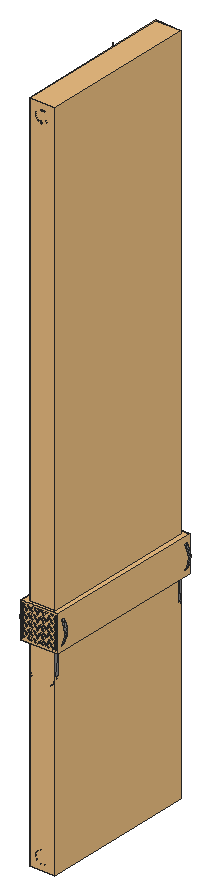
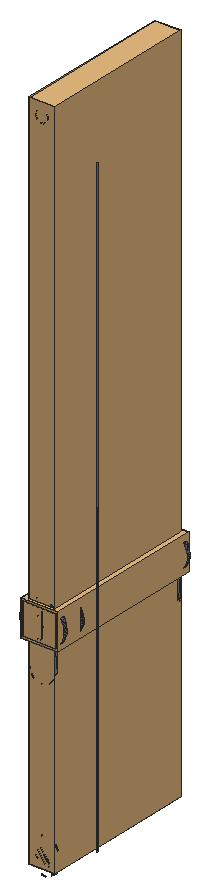
# SketchUp Ruby script. Lengths in inches.
U = 1.inch
M = Sketchup.active_model
def pt(a) = Geom::Point3d.new(a.map { |v| v * U })
def face(e, loops, mat)
  f = e.add_face(loops[0].map { |a| pt(a) })
  loops[1..].each { |l| e.add_face(l.map { |a| pt(a) }).erase! }
  f.material = f.back_material = mat if mat
  f
end
# faces: each face lists its corners as indices into pts; further lists are holes
def faces(e, pts, list, mat = nil) = list.each { |f| face(e, (f[0].is_a?(Array) ? f : [f]).map { |l| l.map { |i| pts[i] } }, mat) }
# xy, xz, yz: faces in a plane at the given z, y or x. An outline is a flat list of corners, or four numbers for a rectangle; further outlines are holes
def ring(l) = l.size == 4 ? [[l[0], l[1]], [l[2], l[1]], [l[2], l[3]], [l[0], l[3]]] : l.each_slice(2).to_a
def flat(e, list, mat, &to3) = list.each { |f| face(e, (f[0].is_a?(Array) ? f : [f]).map { |l| ring(l).map { |u, v| to3.(u, v) } }, mat) }
def xy(e, z, list, mat = nil) = flat(e, list, mat) { |x, y| [x, y, z] }
def xz(e, y, list, mat = nil) = flat(e, list, mat) { |x, z| [x, y, z] }
def yz(e, x, list, mat = nil) = flat(e, list, mat) { |y, z| [x, y, z] }
def lines(e, pts, list) = list.each { |a, b| e.add_line(pt(pts[a]), pt(pts[b])) }
# prism: a flat outline (further loops are holes) pulled along v
def prism(e, loops, v, mat = nil)
  f = face(e, loops, mat); d = Geom::Vector3d.new(v.map { |x| x * U })
  f.pushpull(f.normal.samedirection?(d) ? d.length : -d.length)
end
def box(e, o, s, mat = nil) = prism(e, [[o, [o[0] + s[0], o[1], o[2]], [o[0] + s[0], o[1] + s[1], o[2]], [o[0], o[1] + s[1], o[2]]]], [0, 0, s[2]], mat)
def at(x, y, z, deg = 0) = Geom::Transformation.translation(pt([x, y, z])) * Geom::Transformation.rotation(ORIGIN, Z_AXIS, deg.degrees)
def axes(o, x, y, z) = Geom::Transformation.new([*x, 0, *y, 0, *z, 0, *pt(o).to_a, 1])
def part(name) = M.definitions.add(name)
# library, detail: a bought-in or finely detailed component or shape, given as its bounding box
def library(name, o, s) = part(name).tap { |d| box(d.entities, o, s) }
def detail(e, o, s) = box(e.add_group.entities, o, s)
def put(e, d, t, mat = nil) = e.add_instance(d, t).tap { |i| i.material = mat if mat }
def group(e, t, mat = nil) = e.add_group.tap { |g| g.transformation = t; g.material = mat if mat }.entities
root = M.entities
M.materials.add("Material \#1").color = [140, 140, 140]
c1 = library("3DGeom~4_Defintion",[-18.02,-499.97,-221.16],[36.04,1000,262.12])
c2 = part("3DGeom~5_Defintion")
xy(c2.entities,-225.24,[[-0.79,-499.98,-2.33,-499.64,7.45,-496.14],[-0.79,-499.98,7.45,-496.14,1.58,-499.88],[1.58,-499.88,7.45,-496.14,3.84,-499.16],[-2.33,-499.64,7.4,-485.75,7.45,-496.14],[3.84,-499.16,7.45,-496.14,5.85,-497.89],
  [7.45,-496.14,7.4,-485.75,8.24,-487.08],[7.45,-496.14,8.24,-487.08,8.96,-489.34],[7.45,-496.14,8.96,-489.34,9.0625,-491.71],[7.45,-496.14,9.0625,-491.71,8.55,-494.03],[-7.4,-496.08,-8.24,-494.76,2.32,-482.2],
  [-8.24,-494.76,-8.96,-492.5,2.32,-482.2],[-8.96,-492.5,-9.0625,-490.125,2.32,-482.2],[-9.0625,-490.125,-8.55,-487.81,2.32,-482.2],[-8.55,-487.81,-7.45,-485.7,2.32,-482.2],[-7.45,-485.7,-5.85,-483.95,2.32,-482.2],
  [-5.85,-483.95,-3.84,-482.68,2.32,-482.2],[-3.84,-482.68,-1.58,-481.96,2.32,-482.2],[2.32,-482.2,-1.58,-481.96,0.79,-481.86],[0,481.82,-2.35,482.13,-6.92,496.71],[0,481.82,-6.92,496.71,1.55,482.04],
  [-2.35,482.13,-4.55,483.04,-6.92,496.71],[-4.55,483.04,-6.43,484.49,-6.92,496.71],[-6.43,484.49,-7.88,486.37,-6.92,496.71],[6.92,485.12,-1.55,499.8125,7.88,495.47],[6.92,485.12,7.88,495.47,7.88,486.37],
  [-7.88,486.37,-8.79,488.57,-6.92,496.71],[7.88,486.37,7.88,495.47,8.79,488.57],[-8.79,488.57,-9.1,490.92,-6.92,496.71],[8.79,488.57,7.88,495.47,9.1,490.92],[-9.1,490.92,-8.79,493.28,-6.92,496.71],
  [9.1,490.92,7.88,495.47,8.79,493.28],[-8.79,493.28,-7.88,495.47,-6.92,496.71],[7.88,495.47,-1.55,499.8125,0,500.02],[7.88,495.47,0,500.02,2.35,499.71],[7.88,495.47,2.35,499.71,4.55,498.8],
  [7.88,495.47,4.55,498.8,6.43,497.35]],"Material \#1")
xy(c2.entities,-221.57,[[-2.33,-499.64,-5.22,-498.37,7.4,-485.75],[-5.22,-498.37,-7.4,-496.08,5.22,-483.47],[-5.22,-498.37,5.22,-483.47,7.4,-485.75],[-7.4,-496.08,2.32,-482.2,5.22,-483.47],[1.55,482.04,-6.92,496.71,-4.55,498.8],
  [1.55,482.04,-4.55,498.8,4.55,483.04],[4.55,483.04,-4.55,498.8,-1.55,499.8125],[4.55,483.04,-1.55,499.8125,6.92,485.12]],"Material \#1")
xy(c2.entities,38.05,[[-2.33,-499.64,7.4,-485.75,-5.22,-498.37],[-5.22,-498.37,5.22,-483.47,-7.4,-496.08],[-5.22,-498.37,7.4,-485.75,5.22,-483.47],[-7.4,-496.08,5.22,-483.47,2.32,-482.2],[1.55,482.04,-4.55,498.8,-6.92,496.71],
  [1.55,482.04,4.55,483.04,-4.55,498.8],[4.55,483.04,-1.55,499.8125,-4.55,498.8],[4.55,483.04,6.92,485.12,-1.55,499.8125]],"Material \#1")
xy(c2.entities,41.72,[[-0.79,-499.98,7.45,-496.14,-2.33,-499.64],[-0.79,-499.98,1.58,-499.88,7.45,-496.14],[1.58,-499.88,3.84,-499.16,7.45,-496.14],[-2.33,-499.64,7.45,-496.14,7.4,-485.75],[3.84,-499.16,5.85,-497.89,7.45,-496.14],
  [7.45,-496.14,8.24,-487.08,7.4,-485.75],[7.45,-496.14,8.55,-494.03,9.0625,-491.71],[7.45,-496.14,8.96,-489.34,8.24,-487.08],[7.45,-496.14,9.0625,-491.71,8.96,-489.34],[-7.4,-496.08,2.32,-482.2,-8.24,-494.76],
  [-8.24,-494.76,2.32,-482.2,-8.96,-492.5],[-8.96,-492.5,2.32,-482.2,-9.0625,-490.125],[-9.0625,-490.125,2.32,-482.2,-8.55,-487.81],[-8.55,-487.81,2.32,-482.2,-7.45,-485.7],[-7.45,-485.7,2.32,-482.2,-5.85,-483.95],
  [-5.85,-483.95,2.32,-482.2,-3.84,-482.68],[-3.84,-482.68,2.32,-482.2,-1.58,-481.96],[2.32,-482.2,0.79,-481.86,-1.58,-481.96],[0,481.82,-6.92,496.71,-2.35,482.13],[0,481.82,1.55,482.04,-6.92,496.71],
  [-2.35,482.13,-6.92,496.71,-4.55,483.04],[-4.55,483.04,-6.92,496.71,-6.43,484.49],[-6.43,484.49,-6.92,496.71,-7.88,486.37],[6.92,485.12,7.88,495.47,-1.55,499.8125],[6.92,485.12,7.88,486.37,7.88,495.47],
  [-7.88,486.37,-6.92,496.71,-8.79,488.57],[7.88,486.37,8.79,488.57,7.88,495.47],[-8.79,488.57,-6.92,496.71,-9.1,490.92],[8.79,488.57,9.1,490.92,7.88,495.47],[-9.1,490.92,-6.92,496.71,-8.79,493.28],
  [9.1,490.92,8.79,493.28,7.88,495.47],[-8.79,493.28,-6.92,496.71,-7.88,495.47],[7.88,495.47,0,500.02,-1.55,499.8125],[7.88,495.47,2.35,499.71,0,500.02],[7.88,495.47,4.55,498.8,2.35,499.71],
  [7.88,495.47,6.43,497.35,4.55,498.8]],"Material \#1")
c3 = part("3DGeom~10_Defintion")
yz(c3.entities,-68.96,[[-797.08,-844.83,-797.08,-827.59,-922.41,-827.59],[-922.41,-844.83,-797.08,-844.83,-922.41,-827.59]],"Material \#1")
yz(c3.entities,68.97,[[-922.41,-844.83,-797.08,-827.59,-797.08,-844.83],[-922.41,-844.83,-922.41,-827.59,-797.08,-827.59],[-797.08,137.93,-922.41,155.17,-797.08,155.17],[-922.41,137.93,-922.41,155.17,-797.08,137.93]],"Material \#1")
p = [[-15.8,-989.55,-844.83],[-15.8,-989.55,-827.59],[0,-991.38,-827.59],[0,-991.38,-844.83],[15.8,-989.55,-827.59],[15.8,-989.55,-844.83],
  [-30.32,-984.36,-844.83],[-30.32,-984.36,-827.59],[30.31,-984.36,-827.59],[30.31,-984.36,-844.83],[-43.12,-976.21,-844.83],[-43.12,-976.21,-827.59],
  [43.12,-976.21,-827.59],[43.12,-976.21,-844.83],[-53.81,-965.53,-844.83],[-53.81,-965.53,-827.59],[53.8,-965.53,-827.59],[53.8,-965.53,-844.83],
  [-61.95,-952.73,-844.83],[-61.95,-952.73,-827.59],[53.8,-965.53,-827.59],[61.95,-952.73,-827.59],[61.95,-952.73,-844.83],[-67.15,-938.21,-844.83],
  [-67.15,-938.21,-827.59],[67.14,-938.21,-827.59],[67.14,-938.21,-844.83],[-68.96,-922.41,-844.83],[-68.96,-922.41,-827.59],[67.14,-938.21,-827.59],
  [68.97,-922.41,-827.59],[68.97,-922.41,-844.83],[-69.1,-794.86,-844.83],[-69.1,-794.86,-827.59],[-68.96,-797.08,-827.59],[-68.96,-797.08,-844.83],
  [68.97,-797.08,-844.83],[68.97,-797.08,-827.59],[69.11,-794.71,-827.59],[69.11,-794.71,-844.83],[-69.48,-792.73,-844.83],[-69.48,-792.73,-827.59],
  [69.53,-792.51,-827.59],[69.53,-792.51,-844.83],[-70.14,-790.6875,-844.83],[-70.14,-790.6875,-827.59],[70.24,-790.48,-827.59],[70.24,-790.48,-844.83],
  [-71.08,-788.73,-844.83],[-71.08,-788.73,-827.59],[71.22,-788.57,-827.59],[71.22,-788.57,-844.83],[-72.32,-786.86,-844.83],[-72.32,-786.86,-827.59],
  [72.47,-786.78,-827.59],[72.47,-786.78,-844.83],[-73.8,-785.17,-844.83],[-73.8,-785.17,-827.59],[74,-785.04,-827.59],[74,-785.04,-844.83],
  [-75.96,-783.21,-844.83],[-75.96,-783.21,-827.59],[74,-785.04,-827.59],[75.76,-783.39,-827.59],[75.76,-783.39,-844.83],[86.625,-772.95,-827.59],
  [86.61,-772.96,-844.83],[-86.89,-773.25,-844.83],[-86.89,-773.25,-827.59],[-75.96,-783.21,-844.83],[-96.66,-761.8,-844.83],[-96.66,-761.8,-827.59],
  [86.625,-772.95,-827.59],[86.63,-772.94,-844.83],[86.61,-772.96,-844.83],[86.625,-772.95,-827.59],[86.62,-772.95,-827.59],[86.62,-772.95,-827.59],
  [96.31,-761.375,-827.59],[96.31,-761.375,-844.83],[86.63,-772.94,-844.83],[86.625,-772.95,-827.59],[86.62,-772.95,-827.59],[-104.96,-749.18,-844.83],
  [-104.96,-749.18,-827.59],[-96.66,-761.8,-827.59],[-96.66,-761.8,-844.83],[96.31,-761.375,-827.59],[104.62,-748.77,-827.59],[104.62,-748.77,-844.83],
  [-111.64,-735.52,-844.83],[-111.64,-735.52,-827.59],[111.39,-735.21,-827.59],[111.39,-735.21,-844.83],[-116.49,-721.23,-844.83],[-116.49,-721.23,-827.59],
  [116.4375,-720.78,-827.59],[116.4375,-720.78,-844.83],[-119.64,-705.62,-844.83],[-119.64,-705.62,-827.59],[119.6,-705.57,-827.59],[119.6,-705.57,-844.83],
  [-120.6875,-689.65,-844.83],[-120.6875,-689.65,-827.59],[120.69,-689.65,-827.59],[120.69,-689.65,-844.83],[-117.5,-662,-844.83],[-117.5,-662,-827.59],
  [117.5,-662,-827.59],[117.5,-662,-844.83],[-108.41,-636.61,-844.83],[-108.41,-636.61,-827.59],[117.5,-662,-844.83],[108.41,-636.61,-827.59],
  [108.41,-636.61,-844.83],[-93.91,-613.95,-844.83],[-93.91,-613.95,-827.59],[-108.41,-636.61,-827.59],[108.41,-636.61,-844.83],[94.16,-614.19,-827.59],
  [94.16,-614.19,-844.83],[94.16,-614.19,-827.59],[75.46,-595.5,-827.59],[75.46,-595.5,-844.83],[-75.46,-595.5,-844.83],[-75.46,-595.5,-827.59],
  [-93.91,-613.95,-827.59],[-93.91,-613.95,-827.59],[-93.91,-613.95,-844.83],[-53.05,-581.24,-844.83],[-53.05,-581.24,-827.59],[-75.46,-595.5,-827.59],
  [-75.46,-595.5,-844.83],[53.05,-581.24,-827.59],[53.05,-581.24,-844.83],[-27.65,-572.16,-844.83],[-27.65,-572.16,-827.59],[-53.05,-581.24,-827.59],
  [-53.05,-581.24,-844.83],[27.66,-572.16,-827.59],[27.66,-572.16,-844.83],[0,-568.97,-844.83],[0,-568.97,-827.59],[-27.65,-572.16,-827.59],
  [-27.65,-572.16,-844.83],[0,-568.97,-844.83],[-15.8,-989.55,155.17],[0,-991.38,155.17],[0,-991.38,137.93],[-15.8,-989.55,137.93],
  [15.8,-989.55,155.17],[15.8,-989.55,137.93],[-30.32,-984.36,155.17],[-30.32,-984.36,137.93],[30.31,-984.36,155.17],[30.31,-984.36,137.93],
  [-43.125,-976.22,155.17],[-43.125,-976.22,137.93],[43.12,-976.22,155.17],[43.12,-976.22,137.93],[-53.81,-965.53,155.17],[-53.81,-965.53,137.93],
  [53.8,-965.53,155.17],[53.8,-965.53,137.93],[-61.96,-952.73,155.17],[-61.95,-952.73,137.93],[61.95,-952.73,155.17],[61.95,-952.73,137.93],
  [53.8,-965.53,137.93],[-67.15,-938.21,155.17],[-67.15,-938.21,137.93],[67.14,-938.21,155.17],[67.14,-938.21,137.93],[-68.96,-922.41,155.17],
  [-68.96,-922.41,137.93],[68.97,-922.41,155.17],[68.97,-922.41,137.93],[67.14,-938.21,137.93],[-68.97,-797.08,155.17],[-68.97,-797.08,137.93],
  [-69.1,-794.86,155.17],[-69.1,-794.86,137.93],[68.97,-797.08,155.17],[69.11,-794.71,155.17],[69.11,-794.71,137.93],[68.97,-797.08,137.93],
  [-69.48,-792.73,155.17],[-69.48,-792.73,137.93],[69.53,-792.51,155.17],[69.53,-792.51,137.93],[-70.14,-790.6875,155.17],[-70.14,-790.6875,137.93],
  [70.24,-790.48,155.17],[70.24,-790.48,137.93],[-71.08,-788.73,155.17],[-71.08,-788.73,137.93],[71.22,-788.57,155.17],[71.22,-788.57,137.93],
  [-72.32,-786.86,155.17],[-72.32,-786.86,137.93],[72.47,-786.78,155.17],[72.47,-786.78,137.93],[-73.8,-785.17,155.17],[-73.8,-785.17,137.93],
  [74,-785.04,155.17],[74,-785.04,137.93],[-75.96,-783.21,155.17],[-75.96,-783.21,137.93],[75.76,-783.39,155.17],[75.76,-783.39,137.93],
  [74,-785.04,137.93],[86.61,-772.96,155.17],[86.625,-772.95,137.93],[-86.88,-773.25,155.17],[-75.96,-783.21,155.17],[-86.88,-773.25,137.93],
  [-96.66,-761.8,155.17],[-96.66,-761.8,137.93],[86.63,-772.94,155.17],[86.625,-772.95,137.93],[86.61,-772.96,155.17],[86.62,-772.95,137.93],
  [86.625,-772.95,137.93],[96.31,-761.375,155.17],[96.31,-761.375,137.93],[86.62,-772.95,137.93],[86.63,-772.94,155.17],[86.62,-772.95,137.93],
  [86.625,-772.95,137.93],[-104.96,-749.18,155.17],[-96.66,-761.8,155.17],[-96.66,-761.8,137.93],[-104.96,-749.18,137.93],[104.62,-748.77,155.17],
  [104.62,-748.77,137.93],[96.31,-761.375,137.93],[-111.64,-735.52,155.17],[-111.64,-735.52,137.93],[111.39,-735.21,155.17],[111.39,-735.21,137.93],
  [-116.49,-721.23,155.17],[-116.49,-721.23,137.93],[116.4375,-720.78,155.17],[116.4375,-720.78,137.93],[-119.64,-705.62,155.17],[-119.64,-705.62,137.93],
  [119.6,-705.57,155.17],[119.6,-705.57,137.93],[-120.6875,-689.65,155.17],[-120.6875,-689.65,137.93],[120.69,-689.65,155.17],[120.69,-689.65,137.93],
  [-117.5,-662,155.17],[-117.5,-662,137.93],[117.5,-662,155.17],[117.5,-662,137.93],[-108.41,-636.61,155.17],[-108.41,-636.61,137.93],
  [117.5,-662,155.17],[108.41,-636.61,155.17],[108.41,-636.61,137.93],[-93.91,-613.95,155.17],[-108.41,-636.61,137.93],[-93.91,-613.95,137.93],
  [108.41,-636.61,155.17],[94.16,-614.19,155.17],[94.16,-614.19,137.93],[75.46,-595.5,155.17],[75.46,-595.5,137.93],[94.16,-614.19,137.93],
  [-75.46,-595.5,155.17],[-93.91,-613.95,155.17],[-93.91,-613.95,137.93],[-75.46,-595.5,137.93],[-53.05,-581.24,155.17],[-75.46,-595.5,155.17],
  [-75.46,-595.5,137.93],[-53.05,-581.24,137.93],[53.05,-581.24,155.17],[53.05,-581.24,137.93],[-27.65,-572.16,155.17],[-53.05,-581.24,155.17],
  [-53.05,-581.24,137.93],[-27.65,-572.16,137.93],[27.65,-572.16,155.17],[27.65,-572.16,137.93],[0,-568.97,155.17],[-27.65,-572.16,155.17],
  [-27.65,-572.16,137.93],[0,-568.97,137.93],[0,-568.97,155.17]]
faces(c3.entities,p,[[0,1,2],[2,3,0],[3,2,4],[4,5,3],[6,7,1],[1,0,6],[5,4,8],[8,9,5],
  [10,11,7],[7,6,10],[9,8,12],[12,13,9],[14,15,11],[11,10,14],[13,12,16],[16,17,13],
  [18,19,15],[15,14,18],[17,20,21],[21,22,17],[23,24,19],[19,18,23],[22,21,25],[25,26,22],
  [27,28,24],[24,23,27],[26,29,30],[30,31,26],[32,33,34],[34,35,32],[36,37,38],[38,39,36],
  [40,41,33],[33,32,40],[39,38,42],[42,43,39],[44,45,41],[41,40,44],[43,42,46],[46,47,43],
  [48,49,45],[45,44,48],[47,46,50],[50,51,47],[52,53,49],[49,48,52],[51,50,54],[54,55,51],
  [56,57,53],[53,52,56],[55,54,58],[58,59,55],[60,61,57],[57,56,60],[59,62,63],[63,64,59],
  [64,63,65],[65,66,64],[67,68,61],[61,69,67],[70,71,68],[68,67,70],[72,73,66],[74,75,76],
  [73,77,78],[78,79,73],[80,81,82],[83,84,85],[85,86,83],[79,87,88],[88,89,79],[90,91,84],
  [84,83,90],[89,88,92],[92,93,89],[94,95,91],[91,90,94],[93,92,96],[96,97,93],[98,99,95],
  [95,94,98],[97,96,100],[100,101,97],[102,103,99],[99,98,102],[101,100,104],[104,105,101],[106,107,103],
  [103,102,106],[105,104,108],[108,109,105],[110,111,107],[107,106,110],[112,108,113],[113,114,112],[115,116,117],
  [117,110,115],[118,113,119],[119,120,118],[120,121,122],[122,123,120],[124,125,126],[127,128,124],[129,130,131],
  [131,132,129],[123,122,133],[133,134,123],[135,136,137],[137,138,135],[134,133,139],[139,140,134],[141,142,143],
  [143,144,141],[140,139,142],[142,145,140],[146,147,148],[148,149,146],[147,150,151],[151,148,147],[152,146,149],
  [149,153,152],[150,154,155],[155,151,150],[156,152,153],[153,157,156],[154,158,159],[159,155,154],[160,156,157],
  [157,161,160],[158,162,163],[163,159,158],[164,160,161],[161,165,164],[162,166,167],[167,168,162],[169,164,165],
  [165,170,169],[166,171,172],[172,167,166],[173,169,170],[170,174,173],[171,175,176],[176,177,171],[178,173,174],
  [174,179,178],[180,178,179],[179,181,180],[182,183,184],[184,185,182],[186,180,181],[181,187,186],[183,188,189],
  [189,184,183],[190,186,187],[187,191,190],[188,192,193],[193,189,188],[194,190,191],[191,195,194],[192,196,197],
  [197,193,192],[198,194,195],[195,199,198],[196,200,201],[201,197,196],[202,198,199],[199,203,202],[200,204,205],
  [205,201,200],[206,202,203],[203,207,206],[204,208,209],[209,210,204],[208,211,212],[212,209,208],[213,214,207],
  [207,215,213],[216,213,215],[215,217,216],[211,218,219],[220,221,222],[218,223,224],[224,225,218],[226,227,228],
  [229,230,231],[231,232,229],[223,233,234],[234,235,223],[236,229,232],[232,237,236],[233,238,239],[239,234,233],
  [240,236,237],[237,241,240],[238,242,243],[243,239,238],[244,240,241],[241,245,244],[242,246,247],[247,243,242],
  [248,244,245],[245,249,248],[246,250,251],[251,247,246],[252,248,249],[249,253,252],[250,254,255],[255,251,250],
  [256,252,253],[253,257,256],[258,259,260],[260,255,258],[261,256,262],[262,263,261],[264,265,266],[266,260,264],
  [265,267,268],[268,269,265],[270,271,272],[272,273,270],[274,275,276],[276,277,274],[267,278,279],[279,268,267],
  [280,281,282],[282,283,280],[278,284,285],[285,279,278],[286,287,288],[288,289,286],[284,290,289],[289,285,284]],"Material \#1")
c4 = library("3DGeom~12_Defintion",[-95.68,-755.75,-830.03],[191.36,191.37,1000])
c5 = library("3DGeom~13_Defintion",[-84.91,-744.98,-830.03],[169.82,169.83,1000])
xy(root,190.239,[[338.044,116.355,338.044,116.676,338.08,116.355],[338.08,116.355,338.044,116.676,338.08,116.676]],"Material \#1")
xy(root,190.555,[[338.027,116.355,338.086,116.676,338.027,116.676]],"Material \#1")
xz(root,116.32,[[338.056,189.714,337.988,189.729,338.124,189.729],[338.056,189.714,338.02,189.718,337.988,189.729],[337.988,189.729,337.901,190.151,338.206,189.829],[337.988,189.729,337.906,189.829,337.901,190.151],[337.988,189.729,337.935,189.77,337.906,189.829],
  [337.988,189.729,337.959,189.747,337.935,189.77],[337.935,189.77,337.917,189.798,337.906,189.829],[338.206,189.829,337.898,190.169,337.896,190.174],[338.206,189.829,337.9,190.163,337.898,190.169],[338.206,189.829,337.901,190.157,337.9,190.163],
  [337.906,189.829,337.901,189.864,337.901,190.151],[338.206,189.829,337.901,190.151,337.901,190.157],[338.21,189.864,337.866,190.249,337.903,190.212],[338.21,189.864,337.896,190.174,337.866,190.249],[338.21,189.864,337.903,190.212,337.949,190.184],
  [338.21,189.864,337.949,190.184,338,190.166],[337.896,190.174,337.782,190.362,337.837,190.293],[337.896,190.174,337.892,190.179,337.782,190.362],[337.896,190.174,337.837,190.293,337.866,190.249],[337.892,190.179,337.888,190.184,337.782,190.362],
  [337.888,190.184,337.835,190.237,337.782,190.362],[337.888,190.184,337.882,190.188,337.835,190.237],[337.882,190.188,337.857,190.211,337.835,190.237],[337.835,190.237,337.8,190.295,337.782,190.362],[337.835,190.237,337.816,190.265,337.8,190.295],
  [337.837,190.293,337.782,190.362,337.819,190.343],[337.8,190.295,337.789,190.327,337.782,190.362],[337.819,190.343,337.782,190.362,337.812,190.397],[337.782,190.362,337.78,190.397,337.787,190.459],[337.782,190.362,337.787,190.459,337.84,190.565],
  [337.782,190.362,337.819,190.451,337.812,190.397],[337.782,190.362,337.837,190.501,337.819,190.451],[337.782,190.362,337.84,190.565,337.837,190.501],[337.787,190.459,337.808,190.515,337.84,190.565],[337.837,190.501,337.84,190.565,337.866,190.545],
  [337.866,190.545,337.84,190.565,337.903,190.582],[337.84,190.565,337.883,190.607,337.934,190.638],[337.84,190.565,337.934,190.638,338.056,190.666],[337.84,190.565,337.949,190.61,337.903,190.582],[337.84,190.565,338.056,190.666,337.949,190.61],
  [337.949,190.61,338.056,190.666,338,190.628],[338,190.628,338.056,190.666,338.056,190.634],[337.934,190.638,337.993,190.659,338.056,190.666]],"Material \#1")
xz(root,116.355,[[338.044,190.239,338.068,190.263,338.033,190.263],[338.044,190.239,338.08,190.239,338.068,190.263],[338.033,190.263,338.074,190.271,338.026,190.271],[338.033,190.263,338.068,190.263,338.074,190.271],[338.026,190.271,338.074,190.271,338.074,190.288],
  [338.026,190.271,338.074,190.288,338.026,190.288],[338.026,190.288,338.068,190.296,338.033,190.296],[338.026,190.288,338.074,190.288,338.068,190.296],[338.033,190.296,338.068,190.296,338.08,190.326],[338.033,190.296,338.08,190.326,338.033,190.326],
  [338.033,190.326,338.08,190.326,338.08,190.354],[338.033,190.326,338.08,190.354,338.033,190.354],[338.033,190.354,338.089,190.376,338.024,190.376],[338.033,190.354,338.08,190.354,338.089,190.376],[338.024,190.376,338.089,190.376,338.089,190.398],
  [338.024,190.376,338.089,190.398,338.024,190.398],[338.024,190.398,338.08,190.421,338.033,190.421],[338.024,190.398,338.089,190.398,338.08,190.421],[338.033,190.421,338.086,190.437,338.027,190.437],[338.033,190.421,338.08,190.421,338.086,190.437],
  [338.027,190.437,338.086,190.437,338.086,190.488],[338.027,190.437,338.086,190.488,338.027,190.488],[338.027,190.488,338.078,190.492,338.034,190.492],[338.027,190.488,338.086,190.488,338.078,190.492],[338.034,190.492,338.078,190.492,338.078,190.5],
  [338.034,190.492,338.078,190.5,338.034,190.5],[338.034,190.5,338.086,190.504,338.027,190.504],[338.034,190.5,338.078,190.5,338.086,190.504],[338.027,190.504,338.086,190.504,338.086,190.555],[338.027,190.504,338.086,190.555,338.027,190.555]],"Material \#1")
xz(root,116.597,[[338.056,190.16,338.056,190.168,337.993,190.168],[338.056,190.16,338.117,190.176,338.056,190.168],[338.056,190.16,338.119,190.168,338.117,190.176],[337.993,190.168,337.995,190.176,337.934,190.192],[337.993,190.168,338.056,190.168,337.995,190.176],
  [338.119,190.168,338.174,190.199,338.117,190.176],[338.119,190.168,338.178,190.192,338.174,190.199],[337.995,190.176,337.938,190.199,337.934,190.192],[337.934,190.192,337.938,190.199,337.884,190.23],[338.178,190.192,338.222,190.235,338.174,190.199],
  [338.178,190.192,338.228,190.23,338.222,190.235],[337.938,190.199,337.889,190.235,337.884,190.23],[337.884,190.23,337.889,190.235,337.845,190.279],[338.228,190.23,338.26,190.283,338.222,190.235],[338.228,190.23,338.267,190.279,338.26,190.283],
  [337.889,190.235,337.852,190.283,337.845,190.279],[337.845,190.279,337.852,190.283,337.82,190.336],[338.267,190.279,338.283,190.338,338.26,190.283],[338.267,190.279,338.291,190.336,338.283,190.338],[337.852,190.283,337.828,190.338,337.82,190.336],
  [337.82,190.336,337.828,190.338,337.812,190.397],[338.291,190.336,338.291,190.397,338.283,190.338],[338.291,190.336,338.3,190.397,338.291,190.397],[337.828,190.338,337.82,190.397,337.812,190.397],[337.812,190.397,337.82,190.397,337.82,190.458],
  [337.82,190.397,337.828,190.456,337.82,190.458],[338.291,190.397,338.3,190.397,338.283,190.456],[338.3,190.397,338.291,190.458,338.283,190.456],[337.828,190.456,337.845,190.516,337.82,190.458],[337.828,190.456,337.852,190.512,337.845,190.516],
  [338.283,190.456,338.291,190.458,338.26,190.512],[338.291,190.458,338.267,190.516,338.26,190.512],[337.852,190.512,337.884,190.565,337.845,190.516],[337.852,190.512,337.889,190.559,337.884,190.565],[338.26,190.512,338.267,190.516,338.222,190.559],
  [338.267,190.516,338.228,190.565,338.222,190.559],[337.889,190.559,337.934,190.602,337.884,190.565],[337.889,190.559,337.938,190.595,337.934,190.602],[338.222,190.559,338.228,190.565,338.174,190.595],[338.228,190.565,338.178,190.602,338.174,190.595],
  [337.938,190.595,337.993,190.626,337.934,190.602],[337.938,190.595,337.995,190.618,337.993,190.626],[338.174,190.595,338.178,190.602,338.117,190.618],[338.178,190.602,338.119,190.626,338.117,190.618],[337.995,190.618,338.056,190.634,337.993,190.626],
  [337.995,190.618,338.056,190.626,338.056,190.634],[338.117,190.618,338.119,190.626,338.056,190.626],[338.056,190.626,338.119,190.626,338.056,190.634]],"Material \#1")
xz(root,116.631,[[338.056,187.521,338.056,187.533,338.014,187.525],[337.937,187.553,337.943,187.563,337.904,187.575],[337.943,187.563,337.912,187.584,337.904,187.575],[337.904,187.575,337.912,187.584,337.875,187.603],[337.912,187.584,337.885,187.611,337.875,187.603],
  [337.863,187.861,337.885,187.891,337.875,187.899],[337.885,187.891,337.904,187.926,337.875,187.899],[337.885,187.891,337.912,187.917,337.904,187.926],[337.912,187.917,337.937,187.949,337.904,187.926],[337.912,187.917,337.943,187.939,337.937,187.949],
  [337.943,187.939,337.974,187.966,337.937,187.949],[337.943,187.939,337.978,187.955,337.974,187.966],[337.978,187.955,338.014,187.977,337.974,187.966],[337.978,187.955,338.016,187.965,338.014,187.977],[338.016,187.965,338.056,187.98,338.014,187.977],
  [338.016,187.965,338.056,187.968,338.056,187.98],[337.345,188.032,337.357,188.032,337.345,195.922],[337.357,188.032,337.357,195.922,337.345,195.922]],"Material \#1")
yz(root,338.027,[[116.355,190.504,116.355,190.555,116.676,190.555]],"Material \#1")
yz(root,338.033,[[116.355,190.296,116.355,190.326,116.676,190.326]],"Material \#1")
p = [[337.957,116.624,187.66],[337.977,116.624,187.641],[337.977,116.596,187.641],[337.957,116.596,187.66],[338.002,116.624,187.629],[338.002,116.596,187.629],
  [338.019,116.632,187.654],[338.019,116.604,187.654],[338.076,116.634,187.826],[337.99,116.634,187.706],[337.99,116.607,187.706],[338.076,116.607,187.826],
  [337.974,116.632,187.684],[337.974,116.604,187.684],[338.035,116.634,187.676],[338.035,116.607,187.676],[338.121,116.634,187.795],[338.121,116.607,187.795],
  [338.137,116.632,187.817],[338.137,116.604,187.817],[338.155,116.624,187.842],[338.155,116.596,187.842],[338.135,116.624,187.86],[338.135,116.596,187.86],
  [338.11,116.624,187.873],[338.092,116.632,187.848],[338.092,116.604,187.848],[338.11,116.596,187.873],[338.03,116.676,190.267],[338.044,116.676,190.239],
  [338.044,116.355,190.239],[338.033,116.355,190.263],[338.03,116.676,190.267],[338.03,116.676,190.292],[338.026,116.355,190.288],[338.033,116.355,190.296],
  [338.03,116.676,190.267],[338.033,116.355,190.263],[338.026,116.355,190.271],[338.033,116.355,190.326],[338.033,116.355,190.354],[338.028,116.676,190.365],
  [338.03,116.676,190.292],[338.03,116.676,190.267],[338.026,116.355,190.271],[338.026,116.355,190.288],[338.033,116.676,190.326],[338.03,116.676,190.292],
  [338.033,116.355,190.296],[338.028,116.676,190.365],[338.033,116.676,190.326],[338.033,116.355,190.326],[338.027,116.355,190.437],[338.027,116.355,190.488],
  [338.029,116.676,190.492],[338.033,116.355,190.421],[338.027,116.355,190.437],[338.027,116.676,190.44],[338.024,116.355,190.398],[338.033,116.355,190.421],
  [338.03,116.676,190.429],[338.024,116.355,190.376],[338.024,116.355,190.398],[338.028,116.676,190.41],[338.033,116.355,190.354],[338.024,116.355,190.376],
  [338.024,116.676,190.387],[338.029,116.676,190.492],[338.027,116.676,190.44],[338.027,116.355,190.437],[338.027,116.676,190.44],[338.03,116.676,190.429],
  [338.033,116.355,190.421],[338.03,116.676,190.429],[338.028,116.676,190.41],[338.024,116.355,190.398],[338.028,116.676,190.41],[338.024,116.676,190.387],
  [338.024,116.355,190.376],[338.024,116.676,190.387],[338.028,116.676,190.365],[338.033,116.355,190.354],[338.029,116.676,190.492],[338.034,116.355,190.492],
  [338.034,116.355,190.5],[338.029,116.676,190.492],[338.027,116.355,190.504],[338.029,116.676,190.492],[338.027,116.355,190.488],[338.027,116.676,190.555],
  [338.029,116.676,190.492],[338.027,116.355,190.504],[338.082,116.676,190.498],[338.078,116.355,190.492],[338.086,116.355,190.488],[338.082,116.676,190.498],
  [338.086,116.355,190.504],[338.078,116.355,190.5],[338.082,116.676,190.498]]
faces(root,p,[[0,1,2],[2,3,0],[1,4,5],[5,2,1],[4,6,7],[7,5,4],[8,9,10],[10,11,8],
  [9,12,13],[13,10,9],[12,0,3],[3,13,12],[6,14,15],[15,7,6],[14,16,17],[17,15,14],
  [16,18,19],[19,17,16],[18,20,21],[21,19,18],[20,22,23],[23,21,20],[24,25,26],[26,27,24],
  [25,8,11],[11,26,25],[22,24,27],[27,23,22],[28,29,30],[30,31,32],[33,34,35],[36,37,38],
  [39,40,41],[42,43,44],[44,45,42],[46,47,48],[49,50,51],[52,53,54],[55,56,57],[58,59,60],
  [61,62,63],[64,65,66],[67,68,69],[70,71,72],[73,74,75],[76,77,78],[79,80,81],[82,83,84],
  [85,84,86],[87,88,83],[89,90,91],[92,93,94],[95,96,97],[98,97,93]],"Material \#1")
put(root,c1,axes([338.06,116.32,191.98],[0.00902,0,0],[0,0,0.00877],[0,0.00766,0]),"Material \#1")
put(root,c2,axes([338.06,116.32,191.98],[0.00885,0,0],[0,0,0.00861],[0,0.00752,0]),"Material \#1")
put(root,c3,axes([338.06,116.32,191.98],[0.00236,0,0],[0,0,0.00229],[0,0.002,0]),"Material \#1")
put(root,c4,axes([338.06,116.32,191.98],[0.00246,0,0],[0,0,0.00239],[0,0.00209,0]),"Material \#1")
put(root,c5,axes([338.06,116.32,191.98],[0.00246,0,0],[0,0,0.00239],[0,0.00209,0]),"Material \#1")
